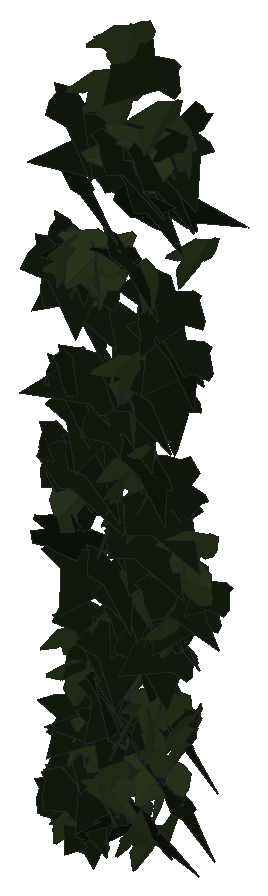
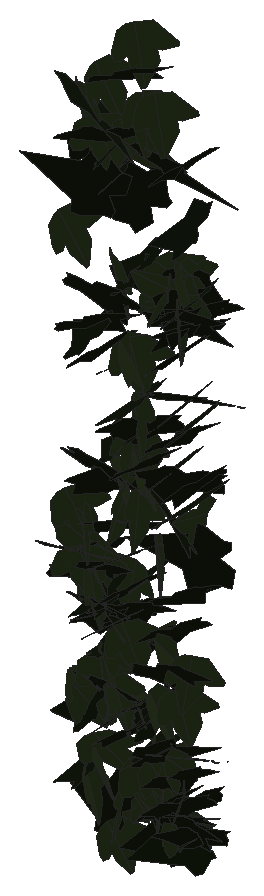
# SketchUp Ruby script. Lengths in inches.
U = 1.inch
M = Sketchup.active_model
def pt(a) = Geom::Point3d.new(a.map { |v| v * U })
def face(e, loops, mat)
  f = e.add_face(loops[0].map { |a| pt(a) })
  loops[1..].each { |l| e.add_face(l.map { |a| pt(a) }).erase! }
  f.material = f.back_material = mat if mat
  f
end
# faces: each face lists its corners as indices into pts; further lists are holes
def faces(e, pts, list, mat = nil) = list.each { |f| face(e, (f[0].is_a?(Array) ? f : [f]).map { |l| l.map { |i| pts[i] } }, mat) }
# xy, xz, yz: faces in a plane at the given z, y or x. An outline is a flat list of corners, or four numbers for a rectangle; further outlines are holes
def ring(l) = l.size == 4 ? [[l[0], l[1]], [l[2], l[1]], [l[2], l[3]], [l[0], l[3]]] : l.each_slice(2).to_a
def flat(e, list, mat, &to3) = list.each { |f| face(e, (f[0].is_a?(Array) ? f : [f]).map { |l| ring(l).map { |u, v| to3.(u, v) } }, mat) }
def xy(e, z, list, mat = nil) = flat(e, list, mat) { |x, y| [x, y, z] }
def xz(e, y, list, mat = nil) = flat(e, list, mat) { |x, z| [x, y, z] }
def yz(e, x, list, mat = nil) = flat(e, list, mat) { |y, z| [x, y, z] }
def lines(e, pts, list) = list.each { |a, b| e.add_line(pt(pts[a]), pt(pts[b])) }
# prism: a flat outline (further loops are holes) pulled along v
def prism(e, loops, v, mat = nil)
  f = face(e, loops, mat); d = Geom::Vector3d.new(v.map { |x| x * U })
  f.pushpull(f.normal.samedirection?(d) ? d.length : -d.length)
end
def box(e, o, s, mat = nil) = prism(e, [[o, [o[0] + s[0], o[1], o[2]], [o[0] + s[0], o[1] + s[1], o[2]], [o[0], o[1] + s[1], o[2]]]], [0, 0, s[2]], mat)
def at(x, y, z, deg = 0) = Geom::Transformation.translation(pt([x, y, z])) * Geom::Transformation.rotation(ORIGIN, Z_AXIS, deg.degrees)
def axes(o, x, y, z) = Geom::Transformation.new([*x, 0, *y, 0, *z, 0, *pt(o).to_a, 1])
def part(name) = M.definitions.add(name)
# library, detail: a bought-in or finely detailed component or shape, given as its bounding box
def library(name, o, s) = part(name).tap { |d| box(d.entities, o, s) }
def detail(e, o, s) = box(e.add_group.entities, o, s)
def put(e, d, t, mat = nil) = e.add_instance(d, t).tap { |i| i.material = mat if mat }
def group(e, t, mat = nil) = e.add_group.tap { |g| g.transformation = t; g.material = mat if mat }.entities
root = M.entities
M.materials.add("1026 AP 7946 SUNNY SIDE UP").color = [254, 231, 186]
M.materials.add("efeu1").color = [18, 25, 13]
M.materials.add("efeu2").color = [43, 57, 29]
c1 = part("ivyleaf_9")
p = [[1.54,2.16,1.25],[1.36,2.04,1.19],[-0.21,0.99,0.68],[-0.71,1.11,0.82],[-0.85,0.86,0.67],[-0.8,0.17,0.21],
  [-0.9,-0.01,0.1],[-0.67,-0.16,-0.02],[-0.08,-0.08,-0.05],[-0.03,-0.6,-0.4],[0.65,-0.88,-0.66],[0.83,-0.6,-0.49],
  [1.29,-0.42,-0.43],[1.8125,-0.07,-0.26],[1.21,0.44,0.15]]
faces(c1.entities,p,[[0,1,2,3,4,5,6,7,8,9,10,11,12,13,14]],"efeu1")
c2 = part("ivyleaf_10")
p = [[0,0.5,-0.03],[-0.0625,2.02,-0.43],[-0.19,2.01,-0.46],[-0.54,1.05,-0.29],[-0.52,0.625,-0.18],[-0.83,0.76,-0.28],
  [-1.16,0.64,-0.33],[-1.15,0.33,-0.24],[-0.77,-0.39,0.02],[-0.3,-0.51,0.16],[0.04,-0.48,0.23],[-0.02,2.01,-0.4375],
  [-0.06,2.01,-0.43],[0.04,-0.49,0.23],[0.67,-0.49,0.14],[1.38,0.36,-0.2],[1.375,0.51,-0.24],[0.81,0.65,-0.19],
  [0.62,0.59,-0.15],[0.6,1.09,-0.28],[0.5,1.23,-0.31]]
faces(c2.entities,p,[[0,1,2,3,4,5,6,7,8,9,10],[11,12,0,13,14,15,16,17,18,19,20]],"efeu2")
put(root,c1,axes([109.18,212.86,275.875],[0.02107,-0.27713,0.10571],[-0.00565,-0.10444,-0.28632],[0.4655,0.01127,-0.00826]),"1026 AP 7946 SUNNY SIDE UP")
put(root,c2,axes([109.35,212.58,270.53],[-0.18385,-0.23941,-0.08467],[0.06528,0.06965,-0.27399],[0.39192,-0.12391,0.00592]),"1026 AP 7946 SUNNY SIDE UP")
put(root,c1,axes([109.25,212.67,275.7],[-0.14356,-0.30674,-0.03698],[0.03696,0.02861,-0.3292],[0.48388,-0.09319,0.01417]),"1026 AP 7946 SUNNY SIDE UP")
put(root,c1,axes([109.53,212.79,275.59],[-0.41233,-0.11188,0.05716],[-0.0641,-0.04684,-0.2927],[0.18608,-0.26404,0.02584]),"1026 AP 7946 SUNNY SIDE UP")
put(root,c2,axes([109.4,212.72,275.64],[0.10376,-0.27297,-0.10119],[0.02112,0.10193,-0.28646],[0.45485,0.05753,0.03639]),"1026 AP 7946 SUNNY SIDE UP")
put(root,c1,axes([109.22,212.67,268.25],[-0.05523,-0.21681,-0.14907],[0.11001,0.13155,-0.22167],[0.39372,-0.06717,0.04103]),"1026 AP 7946 SUNNY SIDE UP")
put(root,c1,axes([109.25,212.59,273.22],[0.03679,-0.28329,-0.05143],[-0.01165,0.04786,-0.29254],[0.45173,0.02431,-0.00336]),"1026 AP 7946 SUNNY SIDE UP")
put(root,c1,axes([109.2,212.47,272.99],[0.22637,-0.21984,-0.1201],[-0.02753,0.12399,-0.26529],[0.38938,0.13657,0.05106]),"1026 AP 7946 SUNNY SIDE UP")
put(root,c1,axes([109.49,212.76,268.42],[-0.39055,-0.06178,-0.06249],[0.10211,-0.01266,-0.26226],[0.08945,-0.25528,0.02654]),"1026 AP 7946 SUNNY SIDE UP")
put(root,c2,axes([109.48,212.64,270.03],[-0.19065,-0.24701,0.0355],[-0.00539,-0.03822,-0.28334],[0.39243,-0.12052,0.01335]),"1026 AP 7946 SUNNY SIDE UP")
put(root,c2,axes([109.47,212.48,276.0625],[-0.00398,-0.28606,0.08594],[0.00595,-0.08507,-0.29517],[0.46922,-0.00135,0.00447]),"1026 AP 7946 SUNNY SIDE UP")
put(root,c1,axes([109.48,212.78,269.3],[-0.34867,-0.15097,0.04916],[0.03729,-0.11413,-0.25455],[0.24657,-0.19622,0.10801]),"1026 AP 7946 SUNNY SIDE UP")
put(root,c1,axes([109.27,212.64,274.06],[0.06096,-0.28152,0.05511],[-0.00052,-0.05564,-0.29297],[0.45106,0.03798,-0.00779]),"1026 AP 7946 SUNNY SIDE UP")
put(root,c1,axes([109.19,212.71,276.93],[0.27366,-0.24878,0.02491],[0.00123,-0.03064,-0.31248],[0.39324,0.17322,-0.01636]),"1026 AP 7946 SUNNY SIDE UP")
put(root,c1,axes([109.29,212.92,275.19],[0.02412,-0.29156,0.01627],[-0.00001,-0.01747,-0.30087],[0.45926,0.01531,-0.00086]),"1026 AP 7946 SUNNY SIDE UP")
put(root,c1,axes([109.34,212.85,268.7],[-0.08747,-0.25278,-0.06632],[0.03253,0.05987,-0.2662],[0.40832,-0.05892,0.007]),"1026 AP 7946 SUNNY SIDE UP")
put(root,c1,axes([109.25,212.64,275.47],[0.04671,-0.26398,-0.1275],[0.07565,0.12567,-0.26674],[0.45114,0.00626,0.05793]),"1026 AP 7946 SUNNY SIDE UP")
put(root,c1,axes([109.33,212.78,277.81],[-0.02122,-0.29946,0.02908],[-0.00326,-0.02987,-0.30899],[0.47321,-0.01363,-0.00082]),"1026 AP 7946 SUNNY SIDE UP")
put(root,c2,axes([109.41,212.69,268.76],[-0.09086,0.18881,-0.17817],[0.04136,-0.17308,-0.20347],[-0.40162,-0.06054,0.01935]),"1026 AP 7946 SUNNY SIDE UP")
put(root,c1,axes([109.4375,212.82,269.05],[-0.1602,-0.24479,0.00768],[0.00341,-0.01048,-0.27314],[0.38515,-0.10173,0.00561]),"1026 AP 7946 SUNNY SIDE UP")
put(root,c1,axes([109.58,212.76,268.4],[-0.33153,-0.1462,0.06342],[-0.00353,-0.10088,-0.25196],[0.24991,-0.19537,0.08056]),"1026 AP 7946 SUNNY SIDE UP")
put(root,c2,axes([109.5,212.72,269.18],[0.00572,-0.16971,0.21169],[0.0744,-0.2028,-0.17378],[0.41359,0.03883,0.02834]),"1026 AP 7946 SUNNY SIDE UP")
put(root,c2,axes([109.58,212.59,268.15],[-0.06732,-0.23257,0.11262],[-0.02794,-0.10922,-0.24425],[0.404,-0.0463,0.00188]),"1026 AP 7946 SUNNY SIDE UP")
put(root,c2,axes([109.5,212.16,272.46],[0.05701,0.06887,-0.29462],[0.09852,0.28013,0.07921],[0.45254,-0.06966,0.01987]),"1026 AP 7946 SUNNY SIDE UP")
put(root,c1,axes([109.19,212.29,272.03],[0.19211,0.10421,-0.23919],[0.24557,0.17347,0.16547],[0.31703,-0.19752,0.01676]),"1026 AP 7946 SUNNY SIDE UP")
put(root,c2,axes([109.25,212.64,275.92],[0.259,-0.06399,0.24625],[0.3592,-0.07218,-0.18222],[0.151,0.28148,0.01109]),"1026 AP 7946 SUNNY SIDE UP")
put(root,c1,axes([109.55,212.68,271.53],[-0.22558,-0.22843,0.08571],[-0.02964,-0.08735,-0.27678],[0.38182,-0.14174,0.02915]),"1026 AP 7946 SUNNY SIDE UP")
put(root,c1,axes([109.64,212.875,270.54],[-0.37051,-0.13521,0.00214],[0.01332,-0.02045,-0.27907],[0.21223,-0.23476,0.02124]),"1026 AP 7946 SUNNY SIDE UP")
put(root,c1,axes([109.59,212.47,275.98],[0.30228,0.21165,-0.09604],[-0.10862,-0.06478,-0.29484],[-0.34786,0.20415,0.00861]),"1026 AP 7946 SUNNY SIDE UP")
put(root,c1,axes([109.52,212.61,267.94],[-0.14438,-0.17967,0.16792],[-0.00265,-0.17484,-0.1993],[0.38252,-0.06903,0.062]),"1026 AP 7946 SUNNY SIDE UP")
put(root,c2,axes([109.5,212.32,268.11],[-0.08276,-0.18114,-0.20364],[0.17268,0.16809,-0.1888],[0.3833,-0.11484,0.04109]),"1026 AP 7946 SUNNY SIDE UP")
put(root,c1,axes([109.4,212.58,274.3125],[0.18834,-0.26181,-0.095],[-0.04298,0.08719,-0.29588],[0.43356,0.12238,0.01193]),"1026 AP 7946 SUNNY SIDE UP")
put(root,c2,axes([109.63,212.53,275.81],[-0.35487,-0.19781,-0.01146],[0.0403,-0.01413,-0.30795],[0.30882,-0.22547,0.02702]),"1026 AP 7946 SUNNY SIDE UP")
put(root,c1,axes([109.42,212.44,267.94],[0.32512,0.07758,0.14485],[0.13611,0.13846,-0.20969],[-0.21196,0.20791,0.08753]),"1026 AP 7946 SUNNY SIDE UP")
put(root,c1,axes([109.84,212.55,274.24],[-0.39373,-0.02955,0.13911],[-0.17056,-0.13167,-0.23738],[0.13514,-0.25228,0.10571]),"1026 AP 7946 SUNNY SIDE UP")
put(root,c1,axes([109.83,212.375,272.45],[-0.03583,0.18086,0.24091],[-0.10126,0.22482,-0.1851],[-0.45238,-0.06465,0.02235]),"1026 AP 7946 SUNNY SIDE UP")
put(root,c1,axes([109.84,212.86,269.2],[-0.21035,-0.05138,0.23219],[-0.28807,-0.13578,-0.14452],[0.22239,-0.22447,0.03241]),"1026 AP 7946 SUNNY SIDE UP")
put(root,c1,axes([109.48,212.42,268.53],[0.02275,-0.27191,-0.12437],[0.00025,0.11933,-0.27975],[0.46682,0.01319,0.00621]),"1026 AP 7946 SUNNY SIDE UP")
put(root,c2,axes([109.7,212.84,270.03],[0.05848,-0.26207,0.04665],[0.00168,-0.04708,-0.2729],[0.41859,0.0368,-0.00542]),"1026 AP 7946 SUNNY SIDE UP")
put(root,c1,axes([109.625,212.59,273.72],[-0.1472,-0.26367,0.08191],[-0.01257,-0.08292,-0.28803],[0.43353,-0.09192,0.01946]),"1026 AP 7946 SUNNY SIDE UP")
put(root,c1,axes([109.58,212.54,268.23],[-0.2403,-0.16594,-0.1388],[0.20428,0.058,-0.22665],[0.26573,-0.19466,0.04872]),"1026 AP 7946 SUNNY SIDE UP")
put(root,c2,axes([109.8,212.5625,276.08],[-0.2285,-0.15522,0.21638],[-0.04239,-0.23107,-0.19567],[0.40959,-0.11051,0.10046]),"1026 AP 7946 SUNNY SIDE UP")
put(root,c2,axes([109.65,212.73,275.84],[-0.05518,0.2593,-0.14995],[-0.00274,-0.14822,-0.26973],[-0.46869,-0.02966,0.01923]),"1026 AP 7946 SUNNY SIDE UP")
put(root,c2,axes([109.79,212.74,268.98],[-0.11113,-0.23589,0.11514],[0.00622,-0.11812,-0.25191],[0.4113,-0.06195,0.03492]),"1026 AP 7946 SUNNY SIDE UP")
put(root,c2,axes([109.8,212.68,278.44],[-0.18479,-0.28512,-0.00217],[0.01051,-0.00223,-0.31763],[0.4482,-0.1175,0.00655]),"1026 AP 7946 SUNNY SIDE UP")
put(root,c1,axes([109.75,212.7,268.46],[-0.16031,-0.22322,0.1428],[-0.05891,-0.13618,-0.2528],[0.41,-0.10685,0.01951]),"1026 AP 7946 SUNNY SIDE UP")
put(root,c2,axes([109.8,212.66,272.125],[0.1338,-0.2458,-0.10902],[0.0013,0.10984,-0.26502],[0.41993,0.07798,0.03556]),"1026 AP 7946 SUNNY SIDE UP")
put(root,c1,axes([110.125,212.51,277.54],[-0.44894,0.07918,0.12293],[-0.19219,0.00202,-0.30381],[-0.11619,-0.30927,0.02755]),"1026 AP 7946 SUNNY SIDE UP")
put(root,c2,axes([109.57,212.52,275.75],[0.26412,0.10364,-0.25336],[0.28143,0.17274,0.20146],[0.31245,-0.24321,0.03272]),"1026 AP 7946 SUNNY SIDE UP")
put(root,c1,axes([109.59,212.43,273.14],[-0.09179,-0.24353,-0.19509],[0.15893,0.16554,-0.25229],[0.45689,-0.10651,0.04857]),"1026 AP 7946 SUNNY SIDE UP")
put(root,c1,axes([109.7,212.55,270.94],[-0.09716,-0.26771,-0.02752],[0.01604,0.0235,-0.28287],[0.42251,-0.06246,0.00441]),"1026 AP 7946 SUNNY SIDE UP")
put(root,c2,axes([109.75,212.64,270.72],[0.10136,-0.19325,0.19482],[0.11324,-0.17629,-0.21069],[0.41105,0.09622,0.01]),"1026 AP 7946 SUNNY SIDE UP")
put(root,c2,axes([109.94,212.79,268.89],[-0.26436,-0.18867,0.09139],[-0.0716,-0.07938,-0.26016],[0.32064,-0.17328,0.01725]),"1026 AP 7946 SUNNY SIDE UP")
put(root,c1,axes([109.65,212.46,273.25],[0.12825,-0.27567,-0.02531],[-0.00948,0.0222,-0.29603],[0.43486,0.08179,0.00101]),"1026 AP 7946 SUNNY SIDE UP")
put(root,c2,axes([109.97,212.39,268.51],[-0.19974,0.17156,0.16122],[-0.16249,0.11674,-0.21894],[-0.32583,-0.16339,0.01035]),"1026 AP 7946 SUNNY SIDE UP")
put(root,c1,axes([109.77,212.3,267.88],[0.13626,0.11555,0.22485],[0.23957,0.15614,-0.14701],[-0.30444,0.17459,-0.01505]),"1026 AP 7946 SUNNY SIDE UP")
put(root,c1,axes([109.85,212.74,269.21],[-0.13459,-0.18846,0.18064],[0.02928,-0.18988,-0.20078],[0.40485,-0.04892,0.07457]),"1026 AP 7946 SUNNY SIDE UP")
put(root,c1,axes([109.86,212.71,269.74],[-0.02901,-0.19747,0.196],[0.00418,-0.19192,-0.20487],[0.43237,-0.01139,0.01513]),"1026 AP 7946 SUNNY SIDE UP")
put(root,c2,axes([109.92,212.51,268.58],[-0.33365,-0.11748,-0.10838],[0.16048,0.03069,-0.24877],[0.18812,-0.23454,0.02]),"1026 AP 7946 SUNNY SIDE UP")
put(root,c2,axes([110.05,212.61,278.34],[-0.16203,-0.28931,-0.03504],[0.03143,0.02723,-0.31607],[0.45667,-0.10452,0.00932]),"1026 AP 7946 SUNNY SIDE UP")
put(root,c1,axes([109.79,212.72,269.69],[0.14302,-0.2113,0.15395],[0.07332,-0.14372,-0.23753],[0.40139,0.10154,-0.01147]),"1026 AP 7946 SUNNY SIDE UP")
put(root,c1,axes([109.98,212.88,273.33],[-0.14764,-0.24365,0.11407],[-0.02429,-0.11367,-0.2685],[0.42102,-0.092,0.02451]),"1026 AP 7946 SUNNY SIDE UP")
put(root,c1,axes([110.08,212.62,269.77],[-0.21764,-0.19012,0.13071],[-0.05656,-0.12961,-0.23923],[0.35588,-0.13687,0.04192]),"1026 AP 7946 SUNNY SIDE UP")
put(root,c2,axes([110.13,212.66,268.85],[-0.09455,-0.25944,0.0159],[0.00961,-0.01876,-0.27427],[0.4087,-0.05958,0.01013]),"1026 AP 7946 SUNNY SIDE UP")
put(root,c2,axes([110.18,212.58,273.98],[0.23901,-0.14668,-0.21037],[-0.0848,0.21313,-0.19864],[0.38506,0.13799,0.08683]),"1026 AP 7946 SUNNY SIDE UP")
put(root,c2,axes([110.13,212.62,272.64],[-0.04972,-0.25899,-0.12781],[0.03799,0.12049,-0.26794],[0.44895,-0.03888,0.00852]),"1026 AP 7946 SUNNY SIDE UP")
put(root,c2,axes([110.16,212.85,270.85],[-0.19895,-0.23188,0.08188],[0.00556,-0.0926,-0.26862],[0.38606,-0.11816,0.04606]),"1026 AP 7946 SUNNY SIDE UP")
put(root,c1,axes([110.09,212.99,274.79],[-0.20871,-0.22137,0.12892],[-0.00053,-0.14235,-0.25804],[0.40082,-0.11545,0.06678]),"1026 AP 7946 SUNNY SIDE UP")
put(root,c1,axes([109.96,212.53,271.69],[0.07853,-0.268,0.04265],[0.00758,-0.04276,-0.28107],[0.4267,0.05008,-0.00286]),"1026 AP 7946 SUNNY SIDE UP")
put(root,c2,axes([110.21,212.57,279.26],[-0.19244,-0.28921,0.00049],[0.0088,-0.00467,-0.32347],[0.45469,-0.12231,0.00647]),"1026 AP 7946 SUNNY SIDE UP")
put(root,c1,axes([110.14,212.53,270.6875],[-0.13977,-0.26749,0.00983],[0.00803,-0.01334,-0.29031],[0.42088,-0.08857,0.0088]),"1026 AP 7946 SUNNY SIDE UP")
put(root,c2,axes([110.26,212.44,273.08],[0.07967,-0.2896,0.0171],[-0.00281,-0.01883,-0.30294],[0.45626,0.05045,-0.00485]),"1026 AP 7946 SUNNY SIDE UP")
put(root,c2,axes([110.52,212.54,277.69],[0.25035,-0.01757,-0.28795],[-0.43982,-0.02362,-0.16281],[-0.01867,0.32072,-0.02587]),"1026 AP 7946 SUNNY SIDE UP")
put(root,c1,axes([110.01,212.73,274.21],[0.20114,-0.25705,-0.06218],[-0.00673,0.06343,-0.29439],[0.4146,0.12573,0.02539]),"1026 AP 7946 SUNNY SIDE UP")
put(root,c1,axes([110.08,212.64,273.81],[-0.09513,-0.26894,-0.12719],[0.07799,0.11344,-0.28246],[0.45772,-0.07522,0.02169]),"1026 AP 7946 SUNNY SIDE UP")
put(root,c2,axes([110.25,212.46,269.62],[0.17695,-0.25834,0.00894],[-0.00816,-0.01332,-0.29018],[0.40644,0.1122,-0.00972]),"1026 AP 7946 SUNNY SIDE UP")
put(root,c1,axes([110.22,212.74,271.14],[-0.18132,-0.23218,0.08942],[-0.04135,-0.08519,-0.2672],[0.3883,-0.11749,0.0133]),"1026 AP 7946 SUNNY SIDE UP")
put(root,c1,axes([110.22,212.86,271.23],[-0.27092,-0.21412,-0.01072],[0.05726,-0.01763,-0.28031],[0.33209,-0.17164,0.03958]),"1026 AP 7946 SUNNY SIDE UP")
put(root,c1,axes([110.32,212.88,278.81],[-0.31708,-0.20521,0.10861],[-0.03312,-0.12454,-0.28879],[0.3621,-0.19109,0.06869]),"1026 AP 7946 SUNNY SIDE UP")
put(root,c1,axes([110.18,212.83,271.48],[-0.07284,-0.26991,0.05215],[0.00065,-0.05296,-0.28228],[0.43226,-0.0454,0.00921]),"1026 AP 7946 SUNNY SIDE UP")
put(root,c1,axes([110.05,212.74,276.04],[0.13586,-0.26541,0.10544],[0.0508,-0.0987,-0.28813],[0.44526,0.09225,0.0007]),"1026 AP 7946 SUNNY SIDE UP")
put(root,c2,axes([110.35,212.48,274.68],[-0.2001,-0.26289,0.04188],[0.00823,-0.04918,-0.3],[0.41857,-0.12471,0.02592]),"1026 AP 7946 SUNNY SIDE UP")
put(root,c2,axes([110.37,212.85,267.93],[-0.0875,-0.25114,0.08224],[-0.01553,-0.081,-0.26536],[0.41476,-0.05602,0.00742]),"1026 AP 7946 SUNNY SIDE UP")
put(root,c1,axes([110.26,212.93,271.92],[-0.17278,-0.22914,0.11216],[0.00466,-0.12116,-0.25728],[0.39975,-0.09763,0.05147]),"1026 AP 7946 SUNNY SIDE UP")
put(root,c1,axes([110.12,212.45,277.74],[0.20708,-0.2699,-0.09187],[-0.03948,0.08516,-0.30854],[0.44446,0.13332,0.0154]),"1026 AP 7946 SUNNY SIDE UP")
put(root,c1,axes([110.17,212.8,269.45],[0.0157,-0.26425,-0.05551],[0.04831,0.05319,-0.2701],[0.42082,0.00375,0.03308]),"1026 AP 7946 SUNNY SIDE UP")
put(root,c2,axes([110.38,212.74,269.93],[-0.00674,-0.27571,0.00472],[0.00498,-0.00619,-0.28408],[0.4336,-0.00422,0.00333]),"1026 AP 7946 SUNNY SIDE UP")
put(root,c2,axes([110.39,212.48,271.52],[-0.39102,0.11373,0.01701],[-0.03926,-0.01661,-0.28058],[-0.17623,-0.24863,0.02476]),"1026 AP 7946 SUNNY SIDE UP")
put(root,c2,axes([110.36,212.5625,274.68],[0.05398,-0.27145,0.11237],[0.03138,-0.10895,-0.28245],[0.45984,0.0393,0.00609]),"1026 AP 7946 SUNNY SIDE UP")
put(root,c2,axes([110.38,212.4,273.37],[-0.16164,-0.26797,-0.09382],[0.07782,0.07674,-0.29465],[0.43739,-0.11268,0.01775]),"1026 AP 7946 SUNNY SIDE UP")
put(root,c2,axes([110.38,212.62,272.55],[-0.00976,-0.20503,-0.21],[0.06326,0.20012,-0.20865],[0.44888,-0.03266,0.02484]),"1026 AP 7946 SUNNY SIDE UP")
put(root,c1,axes([110.18,212.66,271.06],[0.17087,-0.23661,-0.11403],[0.03049,0.12547,-0.25913],[0.40872,0.08956,0.067]),"1026 AP 7946 SUNNY SIDE UP")
put(root,c1,axes([110.05,212.57,276.92],[0.41296,-0.01534,-0.1586],[0.24313,0.02979,0.26899],[0.00299,-0.30292,0.03269]),"1026 AP 7946 SUNNY SIDE UP")
put(root,c2,axes([110.4375,212.43,268.24],[-0.04711,-0.22103,-0.20683],[0.06363,0.19564,-0.22839],[0.46385,-0.04928,0.01033]),"1026 AP 7946 SUNNY SIDE UP")
put(root,c2,axes([110.47,212.63,272.95],[0.17541,-0.26529,-0.02451],[-0.01298,0.02071,-0.29635],[0.4184,0.11186,0.00108]),"1026 AP 7946 SUNNY SIDE UP")
put(root,c1,axes([110.3125,212.86,269.62],[-0.00158,-0.26508,0.04987],[0.00648,-0.04992,-0.27334],[0.42408,-0.00022,0.00436]),"1026 AP 7946 SUNNY SIDE UP")
put(root,c2,axes([110.45,212.71,270.51],[-0.02852,-0.20701,0.19064],[0.0631,-0.18662,-0.21078],[0.43327,0.01355,0.04324]),"1026 AP 7946 SUNNY SIDE UP")
put(root,c2,axes([110.52,212.6,275.87],[0.2701,-0.23562,-0.07003],[-0.0285,0.06894,-0.29886],[0.38396,0.17087,0.02708]),"1026 AP 7946 SUNNY SIDE UP")
put(root,c1,axes([110.79,212.83,271.1],[-0.42454,0.02785,0.03793],[-0.06502,-0.05075,-0.27428],[-0.03184,-0.26771,0.0543]),"1026 AP 7946 SUNNY SIDE UP")
put(root,c1,axes([110.58,212.68,271.13],[-0.25286,0.07458,-0.21817],[0.25589,-0.14149,-0.17911],[-0.24413,-0.22555,0.03823]),"1026 AP 7946 SUNNY SIDE UP")
put(root,c2,axes([110.87,212.33,269.49],[-0.13764,0.07776,0.25137],[-0.39039,0.03565,-0.10344],[-0.09604,-0.25635,0.0602]),"1026 AP 7946 SUNNY SIDE UP")
put(root,c1,axes([110.36,212.63,272.27],[-0.01928,-0.25332,-0.11833],[0.18397,0.09823,-0.23848],[0.39575,-0.05801,0.10509]),"1026 AP 7946 SUNNY SIDE UP")
put(root,c2,axes([110.72,212.67,269.03],[-0.29118,-0.11671,0.15486],[-0.0651,-0.18081,-0.19735],[0.29292,-0.1562,0.11008]),"1026 AP 7946 SUNNY SIDE UP")
put(root,c2,axes([110.7,212.6875,277.84],[-0.31485,-0.22405,0.07101],[-0.00929,-0.08742,-0.30532],[0.36907,-0.19334,0.05289]),"1026 AP 7946 SUNNY SIDE UP")
put(root,c2,axes([110.58,212.86,268.79],[0.23946,-0.20438,0.10072],[0.07275,-0.08869,-0.26265],[0.34955,0.15847,-0.01433]),"1026 AP 7946 SUNNY SIDE UP")
put(root,c1,axes([110.52,212.67,270.49],[-0.08568,-0.20562,0.17977],[0.05732,-0.18314,-0.21027],[0.42136,-0.0169,0.06516]),"1026 AP 7946 SUNNY SIDE UP")
put(root,c1,axes([110.69,212.84,275.63],[-0.40985,-0.10319,-0.08882],[0.14193,0.00339,-0.28726],[0.15592,-0.27434,0.02802]),"1026 AP 7946 SUNNY SIDE UP")
put(root,c1,axes([110.45,212.59,273.33],[0.0741,-0.26649,0.10564],[0.03941,-0.10121,-0.27931],[0.44811,0.05297,0.00709]),"1026 AP 7946 SUNNY SIDE UP")
put(root,c1,axes([110.48,212.48,277.28],[0.22511,-0.26113,-0.06437],[-0.04787,0.05288,-0.30648],[0.41894,0.14636,-0.00043]),"1026 AP 7946 SUNNY SIDE UP")
put(root,c2,axes([110.78,212.57,270.09],[-0.274,-0.1997,0.08909],[-0.04949,-0.08795,-0.27151],[0.33931,-0.17409,0.03235]),"1026 AP 7946 SUNNY SIDE UP")
put(root,c1,axes([110.82,212.71,269.89],[-0.41537,-0.04798,-0.03279],[0.05571,-0.01929,-0.27549],[0.07106,-0.26534,0.02435]),"1026 AP 7946 SUNNY SIDE UP")
put(root,c2,axes([110.67,212.6875,270.24],[0.19316,-0.24023,-0.02261],[0.04699,0.03809,-0.27405],[0.3762,0.11859,0.04584]),"1026 AP 7946 SUNNY SIDE UP")
put(root,c1,axes([110.49,212.69,271.3],[0.2738,-0.21931,-0.03722],[-0.03586,0.02644,-0.28833],[0.34733,0.17561,-0.00043]),"1026 AP 7946 SUNNY SIDE UP")
put(root,c1,axes([110.98,212.75,273.0625],[-0.42584,0.0532,0.0548],[-0.09247,-0.02754,-0.28183],[-0.07324,-0.27456,0.03721]),"1026 AP 7946 SUNNY SIDE UP")
put(root,c2,axes([110.76,212.76,271.36],[0.01043,-0.2803,-0.04084],[0.00027,0.03807,-0.28862],[0.44479,0.00655,0.00113]),"1026 AP 7946 SUNNY SIDE UP")
put(root,c1,axes([110.8125,212.66,270.82],[-0.28801,-0.15287,0.15375],[-0.06601,-0.16806,-0.23006],[0.33035,-0.16686,0.08807]),"1026 AP 7946 SUNNY SIDE UP")
put(root,c1,axes([110.55,212.52,277.65],[0.25201,-0.25587,-0.08805],[-0.07321,0.06998,-0.31062],[0.4171,0.16688,-0.00132]),"1026 AP 7946 SUNNY SIDE UP")
put(root,c1,axes([110.44,212.64,268.15],[0.19841,-0.15284,0.20725],[0.17502,-0.16931,-0.20455],[0.35784,0.16756,-0.01486]),"1026 AP 7946 SUNNY SIDE UP")
put(root,c1,axes([110.59,212.81,277.86],[-0.08741,-0.26184,-0.14634],[0.10859,0.12771,-0.27246],[0.4545,-0.08087,0.03695]),"1026 AP 7946 SUNNY SIDE UP")
put(root,c2,axes([110.74,212.3125,269.75],[0.1299,-0.2113,-0.16386],[0.05832,0.17308,-0.21766],[0.41061,0.04226,0.08275]),"1026 AP 7946 SUNNY SIDE UP")
put(root,c1,axes([110.67,212.5625,270.89],[-0.10939,-0.26868,-0.05565],[0.04433,0.04684,-0.28521],[0.42817,-0.07349,0.01531]),"1026 AP 7946 SUNNY SIDE UP")
put(root,c2,axes([110.86,212.46,278.43],[-0.07349,-0.29438,0.08774],[-0.00019,-0.08782,-0.30728],[0.4826,-0.04487,0.01324]),"1026 AP 7946 SUNNY SIDE UP")
put(root,c2,axes([110.86,212.7,268.48],[0.06613,-0.26651,-0.03021],[0.0004,0.02819,-0.27775],[0.42134,0.0418,0.00501]),"1026 AP 7946 SUNNY SIDE UP")
put(root,c1,axes([111.13,212.54,278.14],[-0.21188,0.26887,0.08243],[-0.11133,0.05157,-0.30692],[-0.42611,-0.14717,0.0392]),"1026 AP 7946 SUNNY SIDE UP")
put(root,c1,axes([110.89,212.79,275.05],[-0.29118,-0.21803,0.07888],[-0.02767,-0.08609,-0.29218],[0.36295,-0.18148,0.041]),"1026 AP 7946 SUNNY SIDE UP")
put(root,c1,axes([110.68,212.54,272.81],[-0.01639,-0.22913,-0.1856],[0.06463,0.17602,-0.23373],[0.45247,-0.03344,0.02666]),"1026 AP 7946 SUNNY SIDE UP")
put(root,c2,axes([110.93,212.79,269.71],[-0.06539,-0.22619,0.14662],[-0.02122,-0.14337,-0.2375],[0.42075,-0.04239,0.01081]),"1026 AP 7946 SUNNY SIDE UP")
put(root,c2,axes([110.92,212.79,271.66],[-0.33469,-0.17718,0.05791],[0.03279,-0.10905,-0.26858],[0.29093,-0.19154,0.0969]),"1026 AP 7946 SUNNY SIDE UP")
put(root,c2,axes([110.96,212.43,271.46],[0.09261,-0.26239,-0.05459],[-0.03189,0.0482,-0.2766],[0.41924,0.06163,-0.00898]),"1026 AP 7946 SUNNY SIDE UP")
put(root,c1,axes([110.99,212.79,271.49],[-0.31578,-0.19518,0.01129],[0.00762,-0.02226,-0.28795],[0.30739,-0.19995,0.01874]),"1026 AP 7946 SUNNY SIDE UP")
put(root,c2,axes([111,212.51,271.26],[-0.04753,-0.27643,0.02185],[0.00045,-0.02294,-0.2866],[0.43614,-0.0301,0.00268]),"1026 AP 7946 SUNNY SIDE UP")
put(root,c2,axes([111.29,212.6,271.86],[-0.0339,0.02245,0.28806],[-0.44021,-0.01725,-0.02092],[0.02441,-0.27979,0.02275]),"1026 AP 7946 SUNNY SIDE UP")
put(root,c1,axes([110.77,212.83,274.86],[0.05765,-0.2406,0.16141],[0.05067,-0.15489,-0.25152],[0.44979,0.04828,0.00765]),"1026 AP 7946 SUNNY SIDE UP")
put(root,c1,axes([110.57,212.77,276.97],[0.20445,-0.06229,0.27617],[0.36711,-0.13277,-0.14902],[0.23017,0.26708,-0.00764]),"1026 AP 7946 SUNNY SIDE UP")
put(root,c1,axes([110.84,212.54,274.57],[-0.02465,-0.2933,0.02799],[0.00117,-0.02891,-0.30275],[0.46341,-0.01553,0.00225]),"1026 AP 7946 SUNNY SIDE UP")
put(root,c2,axes([111.04,212.58,272.14],[0.19278,-0.20833,-0.16506],[-0.03638,0.1663,-0.24181],[0.41052,0.11257,0.05609]),"1026 AP 7946 SUNNY SIDE UP")
put(root,c1,axes([110.75,212.76,269.61],[0.25002,-0.21746,0.06062],[0.03747,-0.0569,-0.27748],[0.35275,0.16017,-0.01349]),"1026 AP 7946 SUNNY SIDE UP")
put(root,c2,axes([111.06,212.71,269.83],[-0.0153,-0.27222,-0.0511],[0.00218,0.04804,-0.28034],[0.43465,-0.00982,-0.00039]),"1026 AP 7946 SUNNY SIDE UP")
put(root,c2,axes([111.11,212.87,276.41],[-0.07057,-0.28022,0.08714],[-0.02452,-0.08478,-0.29284],[0.46033,-0.04747,-0.00224]),"1026 AP 7946 SUNNY SIDE UP")
put(root,c1,axes([110.84,212.68,268.72],[0.22877,-0.22302,-0.01149],[-0.02054,0.00327,-0.27414],[0.35043,0.14579,-0.00857]),"1026 AP 7946 SUNNY SIDE UP")
put(root,c1,axes([111.17,212.86,271.74],[-0.40175,-0.11064,0.01379],[0.04519,-0.09917,-0.26736],[0.16943,-0.23589,0.104]),"1026 AP 7946 SUNNY SIDE UP")
put(root,c1,axes([110.86,212.5,271.74],[0.11239,-0.22885,-0.14554],[0.04781,0.15084,-0.23717],[0.4191,0.04416,0.06609]),"1026 AP 7946 SUNNY SIDE UP")
put(root,c2,axes([111.11,212.53,278.09],[0.29673,-0.22019,-0.10727],[-0.03248,0.11525,-0.29247],[0.38077,0.18142,0.05865]),"1026 AP 7946 SUNNY SIDE UP")
put(root,c2,axes([111.16,212.71,272.36],[-0.17655,-0.2368,0.09734],[-0.02343,-0.09843,-0.26913],[0.40099,-0.11001,0.02713]),"1026 AP 7946 SUNNY SIDE UP")
put(root,c2,axes([111.1,212.6,269.64],[0.03541,-0.23172,0.14222],[0.02656,-0.13837,-0.24063],[0.42435,0.02799,0.00319]),"1026 AP 7946 SUNNY SIDE UP")
